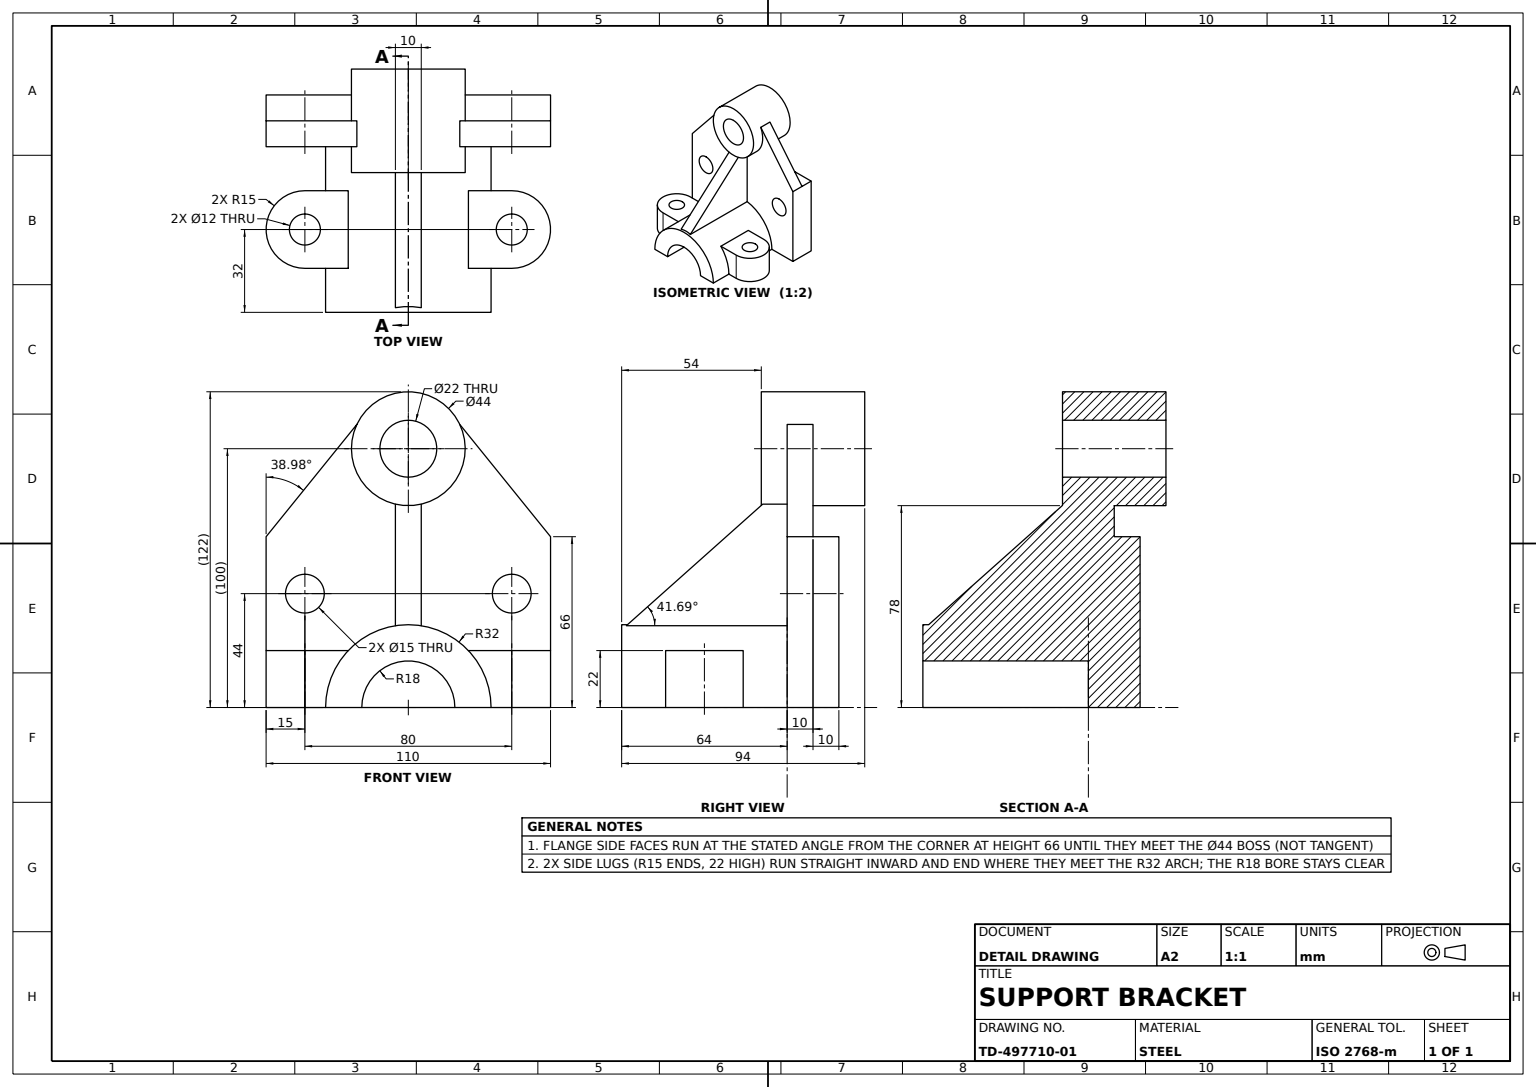
ISO-10303-21;
HEADER;
FILE_DESCRIPTION((''),'2;1');
FILE_NAME('','',(''),(''),'','','');
FILE_SCHEMA(('AUTOMOTIVE_DESIGN'));
ENDSEC;
DATA;
#1=APPLICATION_CONTEXT('');
#2=PRODUCT_CONTEXT('',#1,'mechanical');
#3=PRODUCT('','','',(#2));
#4=PRODUCT_DEFINITION_FORMATION('','',#3);
#5=PRODUCT_DEFINITION_CONTEXT('',#1,'design');
#6=PRODUCT_DEFINITION('','',#4,#5);
#7=PRODUCT_DEFINITION_SHAPE('','',#6);
#8=(LENGTH_UNIT()NAMED_UNIT(*)SI_UNIT(.MILLI.,.METRE.));
#9=(NAMED_UNIT(*)PLANE_ANGLE_UNIT()SI_UNIT($,.RADIAN.));
#10=(NAMED_UNIT(*)SI_UNIT($,.STERADIAN.)SOLID_ANGLE_UNIT());
#11=UNCERTAINTY_MEASURE_WITH_UNIT(LENGTH_MEASURE(0.005),#8,'distance_accuracy_value','');
#12=(GEOMETRIC_REPRESENTATION_CONTEXT(3)GLOBAL_UNCERTAINTY_ASSIGNED_CONTEXT((#11))GLOBAL_UNIT_ASSIGNED_CONTEXT((#8,#9,#10))REPRESENTATION_CONTEXT('',''));
#13=CARTESIAN_POINT('',(-10.,-19.900842,109.378512));
#14=VERTEX_POINT('',#13);
#15=CARTESIAN_POINT('',(-10.,-55.,66.));
#16=VERTEX_POINT('',#15);
#17=CARTESIAN_POINT('',(-10.,-19.5,109.873907));
#18=DIRECTION('',(0.,-0.629016542,-0.777391915));
#19=VECTOR('',#18,1000.);
#20=LINE('',#17,#19);
#21=EDGE_CURVE('',#14,#16,#20,.T.);
#22=ORIENTED_EDGE('',*,*,#21,.T.);
#23=CARTESIAN_POINT('',(0.,-55.,66.));
#24=VERTEX_POINT('',#23);
#25=DIRECTION('',(1.,0.,0.));
#26=VECTOR('',#25,1000.);
#27=LINE('',#15,#26);
#28=EDGE_CURVE('',#16,#24,#27,.T.);
#29=ORIENTED_EDGE('',*,*,#28,.T.);
#30=CARTESIAN_POINT('',(0.,-19.900842,109.378512));
#31=VERTEX_POINT('',#30);
#32=CARTESIAN_POINT('',(0.,-19.5,109.873907));
#33=LINE('',#32,#19);
#34=EDGE_CURVE('',#31,#24,#33,.T.);
#35=ORIENTED_EDGE('',*,*,#34,.F.);
#36=CARTESIAN_POINT('',(10.,-19.900842,109.378512));
#37=DIRECTION('',(-1.,0.,0.));
#38=VECTOR('',#37,1000.);
#39=LINE('',#36,#38);
#40=EDGE_CURVE('',#31,#14,#39,.T.);
#41=ORIENTED_EDGE('',*,*,#40,.T.);
#42=EDGE_LOOP('',(#22,#29,#35,#41));
#43=FACE_BOUND('',#42,.T.);
#44=DIRECTION('',(0.,-0.777391915,0.629016542));
#45=AXIS2_PLACEMENT_3D('',#17,#44,#18);
#46=PLANE('',#45);
#47=ADVANCED_FACE('',(#43),#46,.T.);
#48=CARTESIAN_POINT('',(26.,-40.,22.));
#49=VERTEX_POINT('',#48);
#50=CARTESIAN_POINT('',(32.,-40.,22.));
#51=DIRECTION('',(0.,0.,-1.));
#52=AXIS2_PLACEMENT_3D('',#50,#51,#37);
#53=CIRCLE('',#52,6.);
#54=EDGE_CURVE('',#49,#49,#53,.T.);
#55=ORIENTED_EDGE('',*,*,#54,.T.);
#56=EDGE_LOOP('',(#55));
#57=FACE_BOUND('',#56,.T.);
#58=CARTESIAN_POINT('',(47.,-23.2379,22.));
#59=VERTEX_POINT('',#58);
#60=CARTESIAN_POINT('',(47.,-40.,22.));
#61=VERTEX_POINT('',#60);
#62=CARTESIAN_POINT('',(47.,40.,22.));
#63=DIRECTION('',(0.,-1.,0.));
#64=VECTOR('',#63,1000.);
#65=LINE('',#62,#64);
#66=EDGE_CURVE('',#59,#61,#65,.T.);
#67=ORIENTED_EDGE('',*,*,#66,.F.);
#68=CARTESIAN_POINT('',(17.,-23.2379,22.));
#69=VERTEX_POINT('',#68);
#70=CARTESIAN_POINT('',(64.,-23.2379,22.));
#71=LINE('',#70,#38);
#72=EDGE_CURVE('',#69,#59,#71,.F.);
#73=ORIENTED_EDGE('',*,*,#72,.F.);
#74=CARTESIAN_POINT('',(17.,-40.,22.));
#75=VERTEX_POINT('',#74);
#76=DIRECTION('',(0.,1.,0.));
#77=VECTOR('',#76,1000.);
#78=LINE('',#74,#77);
#79=EDGE_CURVE('',#75,#69,#78,.T.);
#80=ORIENTED_EDGE('',*,*,#79,.F.);
#81=AXIS2_PLACEMENT_3D('',#50,#51,#25);
#82=CIRCLE('',#81,15.);
#83=EDGE_CURVE('',#61,#75,#82,.T.);
#84=ORIENTED_EDGE('',*,*,#83,.F.);
#85=EDGE_LOOP('',(#67,#73,#80,#84));
#86=FACE_BOUND('',#85,.T.);
#87=PLANE('',#52);
#88=ADVANCED_FACE('',(#57,#86),#87,.F.);
#89=CARTESIAN_POINT('',(-20.,-40.,51.5));
#90=VERTEX_POINT('',#89);
#91=CARTESIAN_POINT('',(-20.,-40.,44.));
#92=DIRECTION('',(0.,0.,1.));
#93=AXIS2_PLACEMENT_3D('',#91,#37,#92);
#94=CIRCLE('',#93,7.5);
#95=EDGE_CURVE('',#90,#90,#94,.T.);
#96=ORIENTED_EDGE('',*,*,#95,.T.);
#97=EDGE_LOOP('',(#96));
#98=FACE_BOUND('',#97,.T.);
#99=CARTESIAN_POINT('',(0.,-40.,51.5));
#100=VERTEX_POINT('',#99);
#101=CARTESIAN_POINT('',(0.,-40.,44.));
#102=AXIS2_PLACEMENT_3D('',#101,#37,#92);
#103=CIRCLE('',#102,7.5);
#104=EDGE_CURVE('',#100,#100,#103,.T.);
#105=ORIENTED_EDGE('',*,*,#104,.F.);
#106=EDGE_LOOP('',(#105));
#107=FACE_BOUND('',#106,.T.);
#108=CYLINDRICAL_SURFACE('',#102,7.5);
#109=ADVANCED_FACE('',(#98,#107),#108,.F.);
#110=CARTESIAN_POINT('',(26.,40.,0.));
#111=VERTEX_POINT('',#110);
#112=CARTESIAN_POINT('',(32.,40.,0.));
#113=AXIS2_PLACEMENT_3D('',#112,#51,#37);
#114=CIRCLE('',#113,6.);
#115=EDGE_CURVE('',#111,#111,#114,.T.);
#116=ORIENTED_EDGE('',*,*,#115,.F.);
#117=EDGE_LOOP('',(#116));
#118=FACE_BOUND('',#117,.T.);
#119=CARTESIAN_POINT('',(26.,-40.,0.));
#120=VERTEX_POINT('',#119);
#121=CARTESIAN_POINT('',(32.,-40.,0.));
#122=AXIS2_PLACEMENT_3D('',#121,#51,#37);
#123=CIRCLE('',#122,6.);
#124=EDGE_CURVE('',#120,#120,#123,.T.);
#125=ORIENTED_EDGE('',*,*,#124,.F.);
#126=EDGE_LOOP('',(#125));
#127=FACE_BOUND('',#126,.T.);
#128=CARTESIAN_POINT('',(0.,55.,0.));
#129=VERTEX_POINT('',#128);
#130=CARTESIAN_POINT('',(0.,32.,0.));
#131=VERTEX_POINT('',#130);
#132=LINE('',#128,#64);
#133=EDGE_CURVE('',#129,#131,#132,.T.);
#134=ORIENTED_EDGE('',*,*,#133,.T.);
#135=CARTESIAN_POINT('',(17.,32.,0.));
#136=VERTEX_POINT('',#135);
#137=CARTESIAN_POINT('',(64.,32.,0.));
#138=LINE('',#137,#38);
#139=EDGE_CURVE('',#136,#131,#138,.T.);
#140=ORIENTED_EDGE('',*,*,#139,.F.);
#141=CARTESIAN_POINT('',(17.,40.,0.));
#142=VERTEX_POINT('',#141);
#143=CARTESIAN_POINT('',(17.,-40.,0.));
#144=LINE('',#143,#77);
#145=EDGE_CURVE('',#136,#142,#144,.T.);
#146=ORIENTED_EDGE('',*,*,#145,.T.);
#147=CARTESIAN_POINT('',(47.,40.,0.));
#148=VERTEX_POINT('',#147);
#149=AXIS2_PLACEMENT_3D('',#112,#51,#25);
#150=CIRCLE('',#149,15.);
#151=EDGE_CURVE('',#142,#148,#150,.T.);
#152=ORIENTED_EDGE('',*,*,#151,.T.);
#153=CARTESIAN_POINT('',(47.,32.,0.));
#154=VERTEX_POINT('',#153);
#155=LINE('',#147,#64);
#156=EDGE_CURVE('',#148,#154,#155,.T.);
#157=ORIENTED_EDGE('',*,*,#156,.T.);
#158=VERTEX_POINT('',#137);
#159=EDGE_CURVE('',#158,#154,#138,.T.);
#160=ORIENTED_EDGE('',*,*,#159,.F.);
#161=CARTESIAN_POINT('',(64.,18.,0.));
#162=VERTEX_POINT('',#161);
#163=LINE('',#137,#64);
#164=EDGE_CURVE('',#158,#162,#163,.T.);
#165=ORIENTED_EDGE('',*,*,#164,.T.);
#166=CARTESIAN_POINT('',(0.,18.,0.));
#167=VERTEX_POINT('',#166);
#168=LINE('',#161,#38);
#169=EDGE_CURVE('',#162,#167,#168,.T.);
#170=ORIENTED_EDGE('',*,*,#169,.T.);
#171=CARTESIAN_POINT('',(0.,-18.,0.));
#172=VERTEX_POINT('',#171);
#173=EDGE_CURVE('',#167,#172,#132,.T.);
#174=ORIENTED_EDGE('',*,*,#173,.T.);
#175=CARTESIAN_POINT('',(64.,-18.,0.));
#176=VERTEX_POINT('',#175);
#177=LINE('',#175,#38);
#178=EDGE_CURVE('',#172,#176,#177,.F.);
#179=ORIENTED_EDGE('',*,*,#178,.T.);
#180=CARTESIAN_POINT('',(64.,-32.,0.));
#181=VERTEX_POINT('',#180);
#182=LINE('',#175,#64);
#183=EDGE_CURVE('',#176,#181,#182,.T.);
#184=ORIENTED_EDGE('',*,*,#183,.T.);
#185=CARTESIAN_POINT('',(47.,-32.,0.));
#186=VERTEX_POINT('',#185);
#187=LINE('',#180,#38);
#188=EDGE_CURVE('',#186,#181,#187,.F.);
#189=ORIENTED_EDGE('',*,*,#188,.F.);
#190=CARTESIAN_POINT('',(47.,-40.,0.));
#191=VERTEX_POINT('',#190);
#192=EDGE_CURVE('',#186,#191,#155,.T.);
#193=ORIENTED_EDGE('',*,*,#192,.T.);
#194=VERTEX_POINT('',#143);
#195=AXIS2_PLACEMENT_3D('',#121,#51,#25);
#196=CIRCLE('',#195,15.);
#197=EDGE_CURVE('',#191,#194,#196,.T.);
#198=ORIENTED_EDGE('',*,*,#197,.T.);
#199=CARTESIAN_POINT('',(17.,-32.,0.));
#200=VERTEX_POINT('',#199);
#201=EDGE_CURVE('',#194,#200,#144,.T.);
#202=ORIENTED_EDGE('',*,*,#201,.T.);
#203=CARTESIAN_POINT('',(0.,-32.,0.));
#204=VERTEX_POINT('',#203);
#205=EDGE_CURVE('',#204,#200,#187,.F.);
#206=ORIENTED_EDGE('',*,*,#205,.F.);
#207=CARTESIAN_POINT('',(0.,-55.,0.));
#208=VERTEX_POINT('',#207);
#209=EDGE_CURVE('',#204,#208,#132,.T.);
#210=ORIENTED_EDGE('',*,*,#209,.T.);
#211=CARTESIAN_POINT('',(-20.,-55.,0.));
#212=VERTEX_POINT('',#211);
#213=LINE('',#211,#26);
#214=EDGE_CURVE('',#212,#208,#213,.T.);
#215=ORIENTED_EDGE('',*,*,#214,.F.);
#216=CARTESIAN_POINT('',(-20.,55.,0.));
#217=VERTEX_POINT('',#216);
#218=LINE('',#216,#64);
#219=EDGE_CURVE('',#217,#212,#218,.T.);
#220=ORIENTED_EDGE('',*,*,#219,.F.);
#221=LINE('',#216,#26);
#222=EDGE_CURVE('',#217,#129,#221,.T.);
#223=ORIENTED_EDGE('',*,*,#222,.T.);
#224=EDGE_LOOP('',(#134,#140,#146,#152,#157,#160,#165,#170,#174,#179,#184,#189,#193,#198,#202,#206,#210,#215,#220,#223));
#225=FACE_BOUND('',#224,.T.);
#226=AXIS2_PLACEMENT_3D('',#175,#51,#37);
#227=PLANE('',#226);
#228=ADVANCED_FACE('',(#118,#127,#225),#227,.T.);
#229=ORIENTED_EDGE('',*,*,#145,.F.);
#230=CARTESIAN_POINT('',(17.,23.2379,22.));
#231=VERTEX_POINT('',#230);
#232=CARTESIAN_POINT('',(17.,0.,0.));
#233=AXIS2_PLACEMENT_3D('',#232,#37,#63);
#234=CIRCLE('',#233,32.);
#235=EDGE_CURVE('',#136,#231,#234,.F.);
#236=ORIENTED_EDGE('',*,*,#235,.T.);
#237=CARTESIAN_POINT('',(17.,40.,22.));
#238=VERTEX_POINT('',#237);
#239=EDGE_CURVE('',#231,#238,#78,.T.);
#240=ORIENTED_EDGE('',*,*,#239,.T.);
#241=VECTOR('',#51,1000.);
#242=LINE('',#237,#241);
#243=EDGE_CURVE('',#238,#142,#242,.T.);
#244=ORIENTED_EDGE('',*,*,#243,.T.);
#245=EDGE_LOOP('',(#229,#236,#240,#244));
#246=FACE_BOUND('',#245,.T.);
#247=AXIS2_PLACEMENT_3D('',#74,#37,#63);
#248=PLANE('',#247);
#249=ADVANCED_FACE('',(#246),#248,.T.);
#250=CARTESIAN_POINT('',(-30.,22.,100.));
#251=VERTEX_POINT('',#250);
#252=CARTESIAN_POINT('',(-30.,0.,100.));
#253=AXIS2_PLACEMENT_3D('',#252,#25,#76);
#254=CIRCLE('',#253,22.);
#255=EDGE_CURVE('',#251,#251,#254,.T.);
#256=ORIENTED_EDGE('',*,*,#255,.T.);
#257=EDGE_LOOP('',(#256));
#258=FACE_BOUND('',#257,.T.);
#259=CARTESIAN_POINT('',(0.,5.,78.575715));
#260=VERTEX_POINT('',#259);
#261=CARTESIAN_POINT('',(9.458847,5.,78.575715));
#262=VERTEX_POINT('',#261);
#263=CARTESIAN_POINT('',(10.,5.,78.575715));
#264=LINE('',#263,#38);
#265=EDGE_CURVE('',#260,#262,#264,.F.);
#266=ORIENTED_EDGE('',*,*,#265,.F.);
#267=CARTESIAN_POINT('',(0.,19.900842,109.378512));
#268=VERTEX_POINT('',#267);
#269=CARTESIAN_POINT('',(0.,0.,100.));
#270=AXIS2_PLACEMENT_3D('',#269,#37,#92);
#271=CIRCLE('',#270,22.);
#272=EDGE_CURVE('',#260,#268,#271,.F.);
#273=ORIENTED_EDGE('',*,*,#272,.T.);
#274=CARTESIAN_POINT('',(-10.,19.900842,109.378512));
#275=VERTEX_POINT('',#274);
#276=CARTESIAN_POINT('',(10.,19.900842,109.378512));
#277=LINE('',#276,#38);
#278=EDGE_CURVE('',#275,#268,#277,.F.);
#279=ORIENTED_EDGE('',*,*,#278,.F.);
#280=CARTESIAN_POINT('',(-10.,0.,100.));
#281=AXIS2_PLACEMENT_3D('',#280,#37,#92);
#282=CIRCLE('',#281,22.);
#283=EDGE_CURVE('',#14,#275,#282,.F.);
#284=ORIENTED_EDGE('',*,*,#283,.F.);
#285=ORIENTED_EDGE('',*,*,#40,.F.);
#286=CARTESIAN_POINT('',(0.,-5.,78.575715));
#287=VERTEX_POINT('',#286);
#288=EDGE_CURVE('',#31,#287,#271,.F.);
#289=ORIENTED_EDGE('',*,*,#288,.T.);
#290=CARTESIAN_POINT('',(9.458847,-5.,78.575715));
#291=VERTEX_POINT('',#290);
#292=CARTESIAN_POINT('',(10.,-5.,78.575715));
#293=LINE('',#292,#38);
#294=EDGE_CURVE('',#287,#291,#293,.F.);
#295=ORIENTED_EDGE('',*,*,#294,.T.);
#296=CARTESIAN_POINT('',(10.,-2.028845,78.09375));
#297=VERTEX_POINT('',#296);
#298=CARTESIAN_POINT('',(-14.596491,0.,100.));
#299=DIRECTION('',(-0.66508776,0.,-0.746765205));
#300=DIRECTION('',(-0.746765205,0.,0.66508776));
#301=AXIS2_PLACEMENT_3D('',#298,#299,#300);
#302=ELLIPSE('',#301,33.078341,22.);
#303=EDGE_CURVE('',#297,#291,#302,.T.);
#304=ORIENTED_EDGE('',*,*,#303,.F.);
#305=CARTESIAN_POINT('',(10.,2.028845,78.09375));
#306=VERTEX_POINT('',#305);
#307=CARTESIAN_POINT('',(10.,0.,100.));
#308=AXIS2_PLACEMENT_3D('',#307,#25,#76);
#309=CIRCLE('',#308,22.);
#310=EDGE_CURVE('',#306,#297,#309,.T.);
#311=ORIENTED_EDGE('',*,*,#310,.F.);
#312=EDGE_CURVE('',#262,#306,#302,.T.);
#313=ORIENTED_EDGE('',*,*,#312,.F.);
#314=EDGE_LOOP('',(#266,#273,#279,#284,#285,#289,#295,#304,#311,#313));
#315=FACE_BOUND('',#314,.T.);
#316=AXIS2_PLACEMENT_3D('',#307,#37,#92);
#317=CYLINDRICAL_SURFACE('',#316,22.);
#318=ADVANCED_FACE('',(#258,#315),#317,.T.);
#319=CARTESIAN_POINT('',(0.,40.,51.5));
#320=VERTEX_POINT('',#319);
#321=CARTESIAN_POINT('',(0.,40.,44.));
#322=AXIS2_PLACEMENT_3D('',#321,#37,#92);
#323=CIRCLE('',#322,7.5);
#324=EDGE_CURVE('',#320,#320,#323,.T.);
#325=ORIENTED_EDGE('',*,*,#324,.T.);
#326=EDGE_LOOP('',(#325));
#327=FACE_BOUND('',#326,.T.);
#328=CARTESIAN_POINT('',(0.,55.,66.));
#329=VERTEX_POINT('',#328);
#330=LINE('',#328,#241);
#331=EDGE_CURVE('',#329,#129,#330,.T.);
#332=ORIENTED_EDGE('',*,*,#331,.F.);
#333=DIRECTION('',(0.,-0.629016542,0.777391915));
#334=VECTOR('',#333,1000.);
#335=LINE('',#328,#334);
#336=EDGE_CURVE('',#329,#268,#335,.T.);
#337=ORIENTED_EDGE('',*,*,#336,.T.);
#338=ORIENTED_EDGE('',*,*,#272,.F.);
#339=CARTESIAN_POINT('',(0.,5.,31.606961));
#340=VERTEX_POINT('',#339);
#341=CARTESIAN_POINT('',(0.,5.,87.));
#342=LINE('',#341,#241);
#343=EDGE_CURVE('',#260,#340,#342,.T.);
#344=ORIENTED_EDGE('',*,*,#343,.T.);
#345=CARTESIAN_POINT('',(0.,0.,0.));
#346=AXIS2_PLACEMENT_3D('',#345,#37,#76);
#347=CIRCLE('',#346,32.);
#348=EDGE_CURVE('',#340,#131,#347,.T.);
#349=ORIENTED_EDGE('',*,*,#348,.T.);
#350=ORIENTED_EDGE('',*,*,#133,.F.);
#351=EDGE_LOOP('',(#332,#337,#338,#344,#349,#350));
#352=FACE_BOUND('',#351,.T.);
#353=AXIS2_PLACEMENT_3D('',#345,#37,#92);
#354=PLANE('',#353);
#355=ADVANCED_FACE('',(#327,#352),#354,.F.);
#356=ORIENTED_EDGE('',*,*,#294,.F.);
#357=CARTESIAN_POINT('',(0.,-5.,31.606961));
#358=VERTEX_POINT('',#357);
#359=CARTESIAN_POINT('',(0.,-5.,87.));
#360=LINE('',#359,#241);
#361=EDGE_CURVE('',#287,#358,#360,.T.);
#362=ORIENTED_EDGE('',*,*,#361,.T.);
#363=CARTESIAN_POINT('',(62.195693,-5.,31.606961));
#364=VERTEX_POINT('',#363);
#365=CARTESIAN_POINT('',(64.,-5.,31.606961));
#366=LINE('',#365,#38);
#367=EDGE_CURVE('',#358,#364,#366,.F.);
#368=ORIENTED_EDGE('',*,*,#367,.T.);
#369=CARTESIAN_POINT('',(64.,-5.,30.));
#370=VECTOR('',#300,1000.);
#371=LINE('',#369,#370);
#372=EDGE_CURVE('',#364,#291,#371,.T.);
#373=ORIENTED_EDGE('',*,*,#372,.T.);
#374=EDGE_LOOP('',(#356,#362,#368,#373));
#375=FACE_BOUND('',#374,.T.);
#376=CARTESIAN_POINT('',(0.,-5.,0.));
#377=AXIS2_PLACEMENT_3D('',#376,#63,#51);
#378=PLANE('',#377);
#379=ADVANCED_FACE('',(#375),#378,.T.);
#380=ORIENTED_EDGE('',*,*,#243,.F.);
#381=VERTEX_POINT('',#62);
#382=CARTESIAN_POINT('',(32.,40.,22.));
#383=AXIS2_PLACEMENT_3D('',#382,#51,#25);
#384=CIRCLE('',#383,15.);
#385=EDGE_CURVE('',#238,#381,#384,.T.);
#386=ORIENTED_EDGE('',*,*,#385,.T.);
#387=LINE('',#62,#241);
#388=EDGE_CURVE('',#381,#148,#387,.T.);
#389=ORIENTED_EDGE('',*,*,#388,.T.);
#390=ORIENTED_EDGE('',*,*,#151,.F.);
#391=EDGE_LOOP('',(#380,#386,#389,#390));
#392=FACE_BOUND('',#391,.T.);
#393=AXIS2_PLACEMENT_3D('',#382,#51,#37);
#394=CYLINDRICAL_SURFACE('',#393,15.);
#395=ADVANCED_FACE('',(#392),#394,.T.);
#396=CARTESIAN_POINT('',(64.,0.,0.));
#397=AXIS2_PLACEMENT_3D('',#396,#37,#76);
#398=CIRCLE('',#397,32.);
#399=EDGE_CURVE('',#181,#158,#398,.T.);
#400=ORIENTED_EDGE('',*,*,#399,.F.);
#401=ORIENTED_EDGE('',*,*,#183,.F.);
#402=AXIS2_PLACEMENT_3D('',#396,#25,#76);
#403=CIRCLE('',#402,18.);
#404=EDGE_CURVE('',#162,#176,#403,.T.);
#405=ORIENTED_EDGE('',*,*,#404,.F.);
#406=ORIENTED_EDGE('',*,*,#164,.F.);
#407=EDGE_LOOP('',(#400,#401,#405,#406));
#408=FACE_BOUND('',#407,.T.);
#409=AXIS2_PLACEMENT_3D('',#396,#37,#92);
#410=PLANE('',#409);
#411=ADVANCED_FACE('',(#408),#410,.F.);
#412=ORIENTED_EDGE('',*,*,#79,.T.);
#413=EDGE_CURVE('',#69,#200,#234,.F.);
#414=ORIENTED_EDGE('',*,*,#413,.T.);
#415=ORIENTED_EDGE('',*,*,#201,.F.);
#416=LINE('',#74,#241);
#417=EDGE_CURVE('',#75,#194,#416,.T.);
#418=ORIENTED_EDGE('',*,*,#417,.F.);
#419=EDGE_LOOP('',(#412,#414,#415,#418));
#420=FACE_BOUND('',#419,.T.);
#421=ADVANCED_FACE('',(#420),#248,.T.);
#422=CARTESIAN_POINT('',(47.,23.2379,22.));
#423=VERTEX_POINT('',#422);
#424=CARTESIAN_POINT('',(47.,0.,0.));
#425=AXIS2_PLACEMENT_3D('',#424,#25,#76);
#426=CIRCLE('',#425,32.);
#427=EDGE_CURVE('',#423,#154,#426,.F.);
#428=ORIENTED_EDGE('',*,*,#427,.T.);
#429=ORIENTED_EDGE('',*,*,#156,.F.);
#430=ORIENTED_EDGE('',*,*,#388,.F.);
#431=EDGE_CURVE('',#381,#423,#65,.T.);
#432=ORIENTED_EDGE('',*,*,#431,.T.);
#433=EDGE_LOOP('',(#428,#429,#430,#432));
#434=FACE_BOUND('',#433,.T.);
#435=AXIS2_PLACEMENT_3D('',#62,#25,#76);
#436=PLANE('',#435);
#437=ADVANCED_FACE('',(#434),#436,.T.);
#438=ORIENTED_EDGE('',*,*,#54,.F.);
#439=EDGE_LOOP('',(#438));
#440=FACE_BOUND('',#439,.T.);
#441=ORIENTED_EDGE('',*,*,#124,.T.);
#442=EDGE_LOOP('',(#441));
#443=FACE_BOUND('',#442,.T.);
#444=CYLINDRICAL_SURFACE('',#52,6.);
#445=ADVANCED_FACE('',(#440,#443),#444,.F.);
#446=CARTESIAN_POINT('',(62.195693,5.,31.606961));
#447=VERTEX_POINT('',#446);
#448=CARTESIAN_POINT('',(64.,5.,30.));
#449=LINE('',#448,#370);
#450=EDGE_CURVE('',#447,#262,#449,.T.);
#451=ORIENTED_EDGE('',*,*,#450,.F.);
#452=CARTESIAN_POINT('',(64.,5.,31.606961));
#453=LINE('',#452,#38);
#454=EDGE_CURVE('',#340,#447,#453,.F.);
#455=ORIENTED_EDGE('',*,*,#454,.F.);
#456=ORIENTED_EDGE('',*,*,#343,.F.);
#457=ORIENTED_EDGE('',*,*,#265,.T.);
#458=EDGE_LOOP('',(#451,#455,#456,#457));
#459=FACE_BOUND('',#458,.T.);
#460=CARTESIAN_POINT('',(0.,5.,0.));
#461=AXIS2_PLACEMENT_3D('',#460,#63,#51);
#462=PLANE('',#461);
#463=ADVANCED_FACE('',(#459),#462,.F.);
#464=CARTESIAN_POINT('',(-20.,-55.,66.));
#465=VERTEX_POINT('',#464);
#466=CARTESIAN_POINT('',(-20.,55.,66.));
#467=VERTEX_POINT('',#466);
#468=LINE('',#464,#77);
#469=EDGE_CURVE('',#465,#467,#468,.T.);
#470=ORIENTED_EDGE('',*,*,#469,.T.);
#471=LINE('',#466,#241);
#472=EDGE_CURVE('',#467,#217,#471,.T.);
#473=ORIENTED_EDGE('',*,*,#472,.T.);
#474=ORIENTED_EDGE('',*,*,#219,.T.);
#475=VECTOR('',#92,1000.);
#476=LINE('',#211,#475);
#477=EDGE_CURVE('',#212,#465,#476,.T.);
#478=ORIENTED_EDGE('',*,*,#477,.T.);
#479=EDGE_LOOP('',(#470,#473,#474,#478));
#480=FACE_BOUND('',#479,.T.);
#481=CARTESIAN_POINT('',(-20.,40.,51.5));
#482=VERTEX_POINT('',#481);
#483=CARTESIAN_POINT('',(-20.,40.,44.));
#484=AXIS2_PLACEMENT_3D('',#483,#37,#92);
#485=CIRCLE('',#484,7.5);
#486=EDGE_CURVE('',#482,#482,#485,.T.);
#487=ORIENTED_EDGE('',*,*,#486,.F.);
#488=EDGE_LOOP('',(#487));
#489=FACE_BOUND('',#488,.T.);
#490=ORIENTED_EDGE('',*,*,#95,.F.);
#491=EDGE_LOOP('',(#490));
#492=FACE_BOUND('',#491,.T.);
#493=CARTESIAN_POINT('',(-20.,0.,0.));
#494=AXIS2_PLACEMENT_3D('',#493,#37,#92);
#495=PLANE('',#494);
#496=ADVANCED_FACE('',(#480,#489,#492),#495,.T.);
#497=ORIENTED_EDGE('',*,*,#404,.T.);
#498=ORIENTED_EDGE('',*,*,#178,.F.);
#499=AXIS2_PLACEMENT_3D('',#345,#25,#76);
#500=CIRCLE('',#499,18.);
#501=EDGE_CURVE('',#167,#172,#500,.T.);
#502=ORIENTED_EDGE('',*,*,#501,.F.);
#503=ORIENTED_EDGE('',*,*,#169,.F.);
#504=EDGE_LOOP('',(#497,#498,#502,#503));
#505=FACE_BOUND('',#504,.T.);
#506=CYLINDRICAL_SURFACE('',#409,18.);
#507=ADVANCED_FACE('',(#505),#506,.F.);
#508=CARTESIAN_POINT('',(10.,0.,111.));
#509=VERTEX_POINT('',#508);
#510=CIRCLE('',#316,11.);
#511=EDGE_CURVE('',#509,#509,#510,.T.);
#512=ORIENTED_EDGE('',*,*,#511,.T.);
#513=EDGE_LOOP('',(#512));
#514=FACE_BOUND('',#513,.T.);
#515=CARTESIAN_POINT('',(10.,0.,78.09375));
#516=LINE('',#515,#77);
#517=EDGE_CURVE('',#297,#306,#516,.T.);
#518=ORIENTED_EDGE('',*,*,#517,.T.);
#519=ORIENTED_EDGE('',*,*,#310,.T.);
#520=EDGE_LOOP('',(#518,#519));
#521=FACE_BOUND('',#520,.T.);
#522=AXIS2_PLACEMENT_3D('',#307,#25,#51);
#523=PLANE('',#522);
#524=ADVANCED_FACE('',(#514,#521),#523,.T.);
#525=ORIENTED_EDGE('',*,*,#283,.T.);
#526=CARTESIAN_POINT('',(-10.,55.,66.));
#527=VERTEX_POINT('',#526);
#528=LINE('',#526,#334);
#529=EDGE_CURVE('',#527,#275,#528,.T.);
#530=ORIENTED_EDGE('',*,*,#529,.F.);
#531=LINE('',#15,#77);
#532=EDGE_CURVE('',#16,#527,#531,.T.);
#533=ORIENTED_EDGE('',*,*,#532,.F.);
#534=ORIENTED_EDGE('',*,*,#21,.F.);
#535=EDGE_LOOP('',(#525,#530,#533,#534));
#536=FACE_BOUND('',#535,.T.);
#537=CARTESIAN_POINT('',(-10.,0.,0.));
#538=AXIS2_PLACEMENT_3D('',#537,#37,#92);
#539=PLANE('',#538);
#540=ADVANCED_FACE('',(#536),#539,.T.);
#541=CARTESIAN_POINT('',(26.,40.,22.));
#542=VERTEX_POINT('',#541);
#543=CIRCLE('',#393,6.);
#544=EDGE_CURVE('',#542,#542,#543,.T.);
#545=ORIENTED_EDGE('',*,*,#544,.T.);
#546=EDGE_LOOP('',(#545));
#547=FACE_BOUND('',#546,.T.);
#548=ORIENTED_EDGE('',*,*,#385,.F.);
#549=ORIENTED_EDGE('',*,*,#239,.F.);
#550=CARTESIAN_POINT('',(64.,23.2379,22.));
#551=LINE('',#550,#38);
#552=EDGE_CURVE('',#423,#231,#551,.T.);
#553=ORIENTED_EDGE('',*,*,#552,.F.);
#554=ORIENTED_EDGE('',*,*,#431,.F.);
#555=EDGE_LOOP('',(#548,#549,#553,#554));
#556=FACE_BOUND('',#555,.T.);
#557=ADVANCED_FACE('',(#547,#556),#87,.F.);
#558=ORIENTED_EDGE('',*,*,#288,.F.);
#559=ORIENTED_EDGE('',*,*,#34,.T.);
#560=LINE('',#207,#475);
#561=EDGE_CURVE('',#208,#24,#560,.T.);
#562=ORIENTED_EDGE('',*,*,#561,.F.);
#563=ORIENTED_EDGE('',*,*,#209,.F.);
#564=EDGE_CURVE('',#204,#358,#347,.T.);
#565=ORIENTED_EDGE('',*,*,#564,.T.);
#566=ORIENTED_EDGE('',*,*,#361,.F.);
#567=EDGE_LOOP('',(#558,#559,#562,#563,#565,#566));
#568=FACE_BOUND('',#567,.T.);
#569=ORIENTED_EDGE('',*,*,#104,.T.);
#570=EDGE_LOOP('',(#569));
#571=FACE_BOUND('',#570,.T.);
#572=ADVANCED_FACE('',(#568,#571),#354,.F.);
#573=ORIENTED_EDGE('',*,*,#255,.F.);
#574=EDGE_LOOP('',(#573));
#575=FACE_BOUND('',#574,.T.);
#576=CARTESIAN_POINT('',(-30.,0.,89.));
#577=VERTEX_POINT('',#576);
#578=AXIS2_PLACEMENT_3D('',#252,#25,#51);
#579=CIRCLE('',#578,11.);
#580=EDGE_CURVE('',#577,#577,#579,.T.);
#581=ORIENTED_EDGE('',*,*,#580,.T.);
#582=EDGE_LOOP('',(#581));
#583=FACE_BOUND('',#582,.T.);
#584=PLANE('',#578);
#585=ADVANCED_FACE('',(#575,#583),#584,.F.);
#586=ORIENTED_EDGE('',*,*,#139,.T.);
#587=ORIENTED_EDGE('',*,*,#348,.F.);
#588=ORIENTED_EDGE('',*,*,#454,.T.);
#589=CARTESIAN_POINT('',(97.684211,0.,0.));
#590=AXIS2_PLACEMENT_3D('',#589,#299,#300);
#591=ELLIPSE('',#590,48.113951,32.);
#592=EDGE_CURVE('',#447,#364,#591,.F.);
#593=ORIENTED_EDGE('',*,*,#592,.T.);
#594=ORIENTED_EDGE('',*,*,#367,.F.);
#595=ORIENTED_EDGE('',*,*,#564,.F.);
#596=ORIENTED_EDGE('',*,*,#205,.T.);
#597=ORIENTED_EDGE('',*,*,#413,.F.);
#598=ORIENTED_EDGE('',*,*,#72,.T.);
#599=EDGE_CURVE('',#186,#59,#426,.F.);
#600=ORIENTED_EDGE('',*,*,#599,.F.);
#601=ORIENTED_EDGE('',*,*,#188,.T.);
#602=ORIENTED_EDGE('',*,*,#399,.T.);
#603=ORIENTED_EDGE('',*,*,#159,.T.);
#604=ORIENTED_EDGE('',*,*,#427,.F.);
#605=ORIENTED_EDGE('',*,*,#552,.T.);
#606=ORIENTED_EDGE('',*,*,#235,.F.);
#607=EDGE_LOOP('',(#586,#587,#588,#593,#594,#595,#596,#597,#598,#600,#601,#602,#603,#604,#605,#606));
#608=FACE_BOUND('',#607,.T.);
#609=CYLINDRICAL_SURFACE('',#409,32.);
#610=ADVANCED_FACE('',(#608),#609,.T.);
#611=ORIENTED_EDGE('',*,*,#331,.T.);
#612=ORIENTED_EDGE('',*,*,#222,.F.);
#613=ORIENTED_EDGE('',*,*,#472,.F.);
#614=LINE('',#466,#26);
#615=EDGE_CURVE('',#467,#527,#614,.T.);
#616=ORIENTED_EDGE('',*,*,#615,.T.);
#617=LINE('',#526,#26);
#618=EDGE_CURVE('',#527,#329,#617,.T.);
#619=ORIENTED_EDGE('',*,*,#618,.T.);
#620=EDGE_LOOP('',(#611,#612,#613,#616,#619));
#621=FACE_BOUND('',#620,.T.);
#622=AXIS2_PLACEMENT_3D('',#466,#63,#51);
#623=PLANE('',#622);
#624=ADVANCED_FACE('',(#621),#623,.F.);
#625=ORIENTED_EDGE('',*,*,#618,.F.);
#626=ORIENTED_EDGE('',*,*,#529,.T.);
#627=ORIENTED_EDGE('',*,*,#278,.T.);
#628=ORIENTED_EDGE('',*,*,#336,.F.);
#629=EDGE_LOOP('',(#625,#626,#627,#628));
#630=FACE_BOUND('',#629,.T.);
#631=DIRECTION('',(0.,0.777391915,0.629016542));
#632=AXIS2_PLACEMENT_3D('',#526,#631,#333);
#633=PLANE('',#632);
#634=ADVANCED_FACE('',(#630),#633,.T.);
#635=ORIENTED_EDGE('',*,*,#115,.T.);
#636=EDGE_LOOP('',(#635));
#637=FACE_BOUND('',#636,.T.);
#638=ORIENTED_EDGE('',*,*,#544,.F.);
#639=EDGE_LOOP('',(#638));
#640=FACE_BOUND('',#639,.T.);
#641=CYLINDRICAL_SURFACE('',#393,6.);
#642=ADVANCED_FACE('',(#637,#640),#641,.F.);
#643=ORIENTED_EDGE('',*,*,#312,.T.);
#644=ORIENTED_EDGE('',*,*,#517,.F.);
#645=ORIENTED_EDGE('',*,*,#303,.T.);
#646=ORIENTED_EDGE('',*,*,#372,.F.);
#647=ORIENTED_EDGE('',*,*,#592,.F.);
#648=ORIENTED_EDGE('',*,*,#450,.T.);
#649=EDGE_LOOP('',(#643,#644,#645,#646,#647,#648));
#650=FACE_BOUND('',#649,.T.);
#651=AXIS2_PLACEMENT_3D('',#369,#299,#300);
#652=PLANE('',#651);
#653=ADVANCED_FACE('',(#650),#652,.F.);
#654=ORIENTED_EDGE('',*,*,#28,.F.);
#655=LINE('',#464,#26);
#656=EDGE_CURVE('',#465,#16,#655,.T.);
#657=ORIENTED_EDGE('',*,*,#656,.F.);
#658=ORIENTED_EDGE('',*,*,#477,.F.);
#659=ORIENTED_EDGE('',*,*,#214,.T.);
#660=ORIENTED_EDGE('',*,*,#561,.T.);
#661=EDGE_LOOP('',(#654,#657,#658,#659,#660));
#662=FACE_BOUND('',#661,.T.);
#663=AXIS2_PLACEMENT_3D('',#211,#76,#92);
#664=PLANE('',#663);
#665=ADVANCED_FACE('',(#662),#664,.F.);
#666=ORIENTED_EDGE('',*,*,#580,.F.);
#667=EDGE_LOOP('',(#666));
#668=FACE_BOUND('',#667,.T.);
#669=ORIENTED_EDGE('',*,*,#511,.F.);
#670=EDGE_LOOP('',(#669));
#671=FACE_BOUND('',#670,.T.);
#672=CYLINDRICAL_SURFACE('',#316,11.);
#673=ADVANCED_FACE('',(#668,#671),#672,.F.);
#674=ORIENTED_EDGE('',*,*,#417,.T.);
#675=ORIENTED_EDGE('',*,*,#197,.F.);
#676=LINE('',#60,#241);
#677=EDGE_CURVE('',#61,#191,#676,.T.);
#678=ORIENTED_EDGE('',*,*,#677,.F.);
#679=ORIENTED_EDGE('',*,*,#83,.T.);
#680=EDGE_LOOP('',(#674,#675,#678,#679));
#681=FACE_BOUND('',#680,.T.);
#682=CYLINDRICAL_SURFACE('',#52,15.);
#683=ADVANCED_FACE('',(#681),#682,.T.);
#684=ORIENTED_EDGE('',*,*,#486,.T.);
#685=EDGE_LOOP('',(#684));
#686=FACE_BOUND('',#685,.T.);
#687=ORIENTED_EDGE('',*,*,#324,.F.);
#688=EDGE_LOOP('',(#687));
#689=FACE_BOUND('',#688,.T.);
#690=CYLINDRICAL_SURFACE('',#322,7.5);
#691=ADVANCED_FACE('',(#686,#689),#690,.F.);
#692=ORIENTED_EDGE('',*,*,#501,.T.);
#693=ORIENTED_EDGE('',*,*,#173,.F.);
#694=EDGE_LOOP('',(#692,#693));
#695=FACE_BOUND('',#694,.T.);
#696=ADVANCED_FACE('',(#695),#354,.F.);
#697=ORIENTED_EDGE('',*,*,#66,.T.);
#698=ORIENTED_EDGE('',*,*,#677,.T.);
#699=ORIENTED_EDGE('',*,*,#192,.F.);
#700=ORIENTED_EDGE('',*,*,#599,.T.);
#701=EDGE_LOOP('',(#697,#698,#699,#700));
#702=FACE_BOUND('',#701,.T.);
#703=ADVANCED_FACE('',(#702),#436,.T.);
#704=ORIENTED_EDGE('',*,*,#532,.T.);
#705=ORIENTED_EDGE('',*,*,#615,.F.);
#706=ORIENTED_EDGE('',*,*,#469,.F.);
#707=ORIENTED_EDGE('',*,*,#656,.T.);
#708=EDGE_LOOP('',(#704,#705,#706,#707));
#709=FACE_BOUND('',#708,.T.);
#710=AXIS2_PLACEMENT_3D('',#464,#51,#37);
#711=PLANE('',#710);
#712=ADVANCED_FACE('',(#709),#711,.F.);
#713=CLOSED_SHELL('',(#47,#88,#109,#228,#249,#318,#355,#379,#395,#411,#421,#437,#445,#463,#496,#507,#524,#540,#557,#572,#585,#610,#624,#634,#642,#653,#665,#673,#683,#691,#696,#703,#712));
#714=MANIFOLD_SOLID_BREP('',#713);
#715=ADVANCED_BREP_SHAPE_REPRESENTATION('',(#714),#12);
#716=SHAPE_DEFINITION_REPRESENTATION(#7,#715);
ENDSEC;
END-ISO-10303-21;
